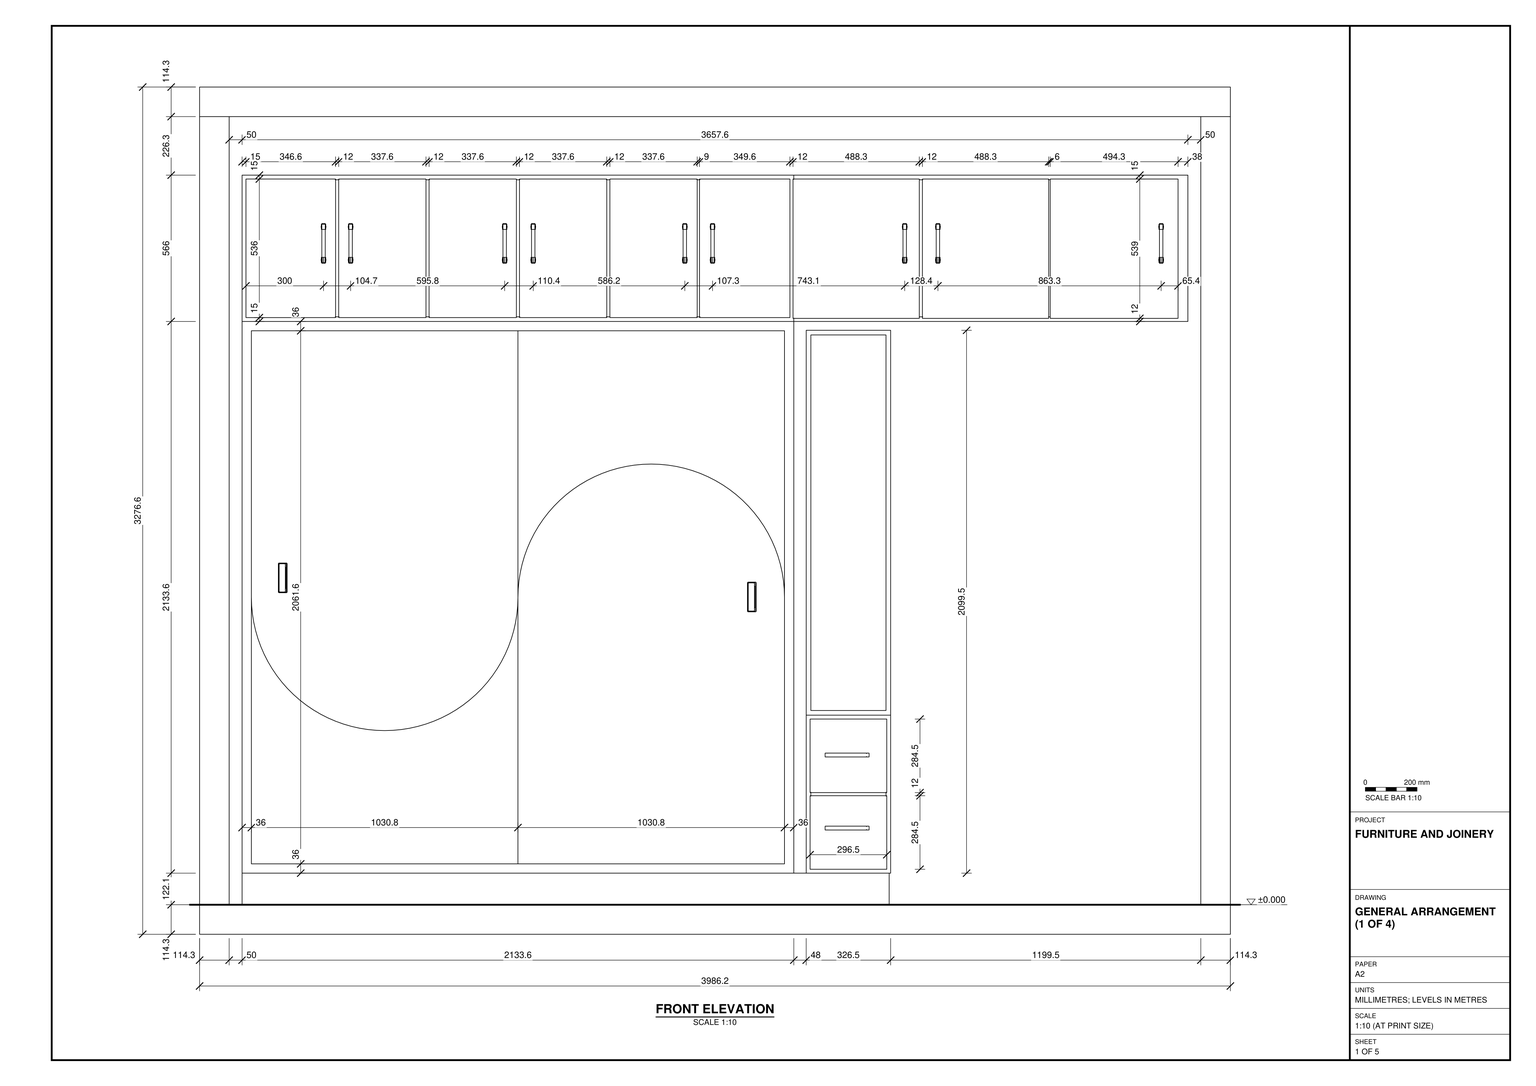
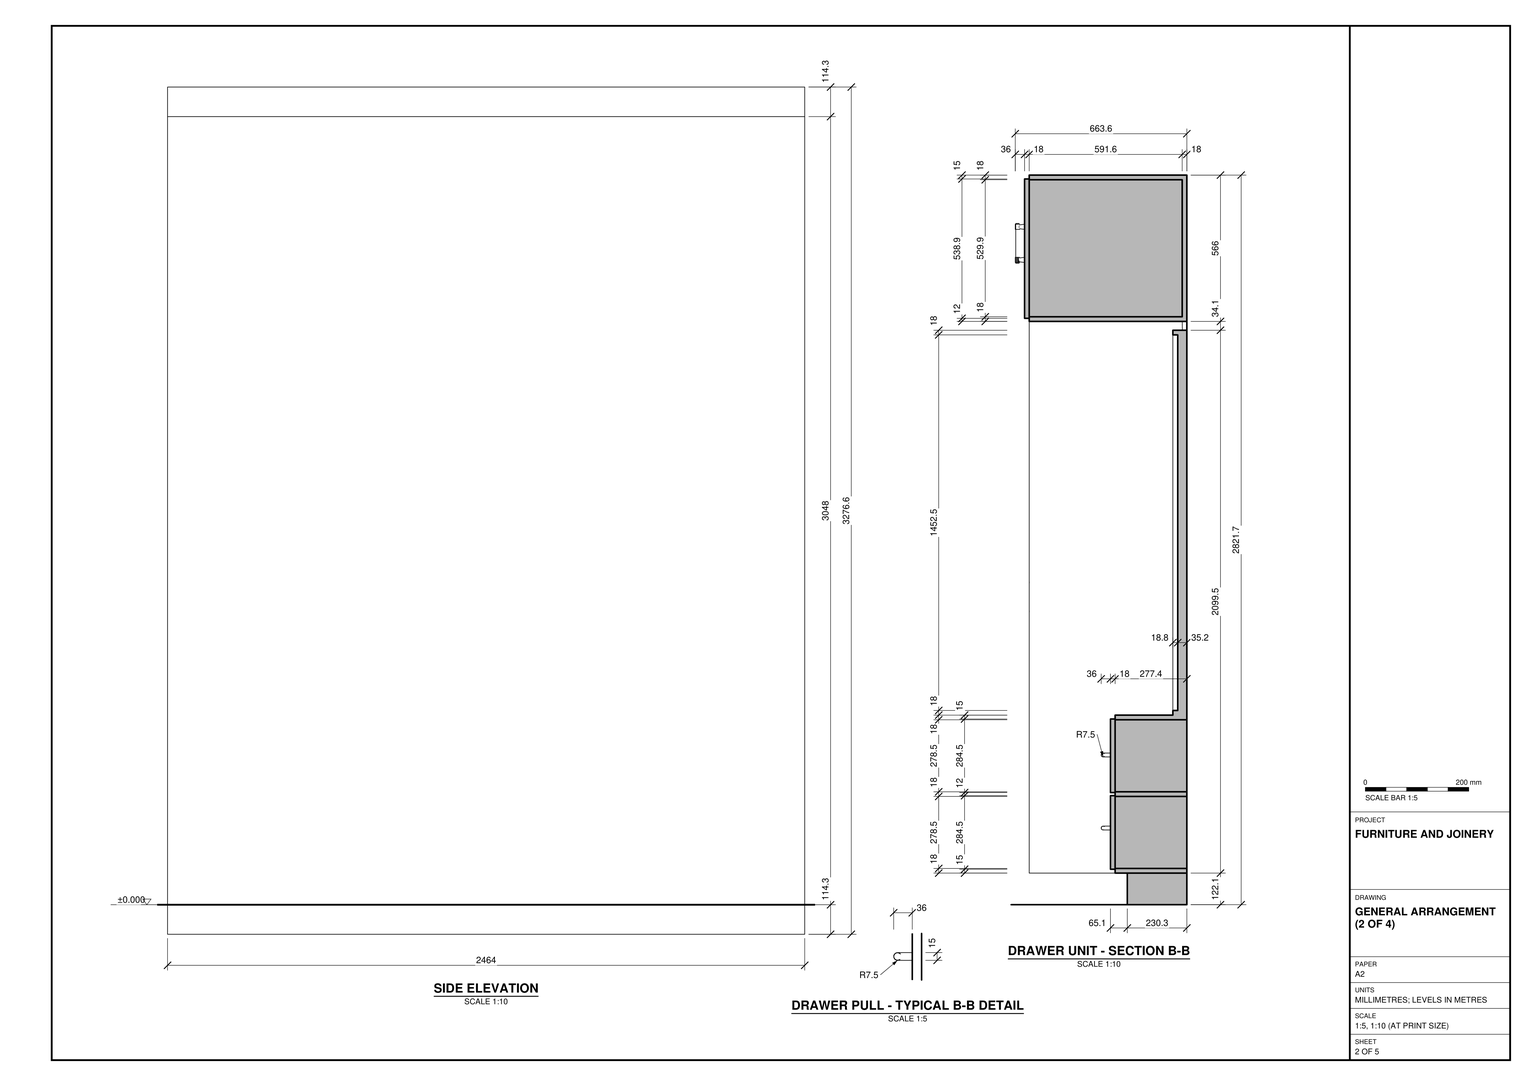
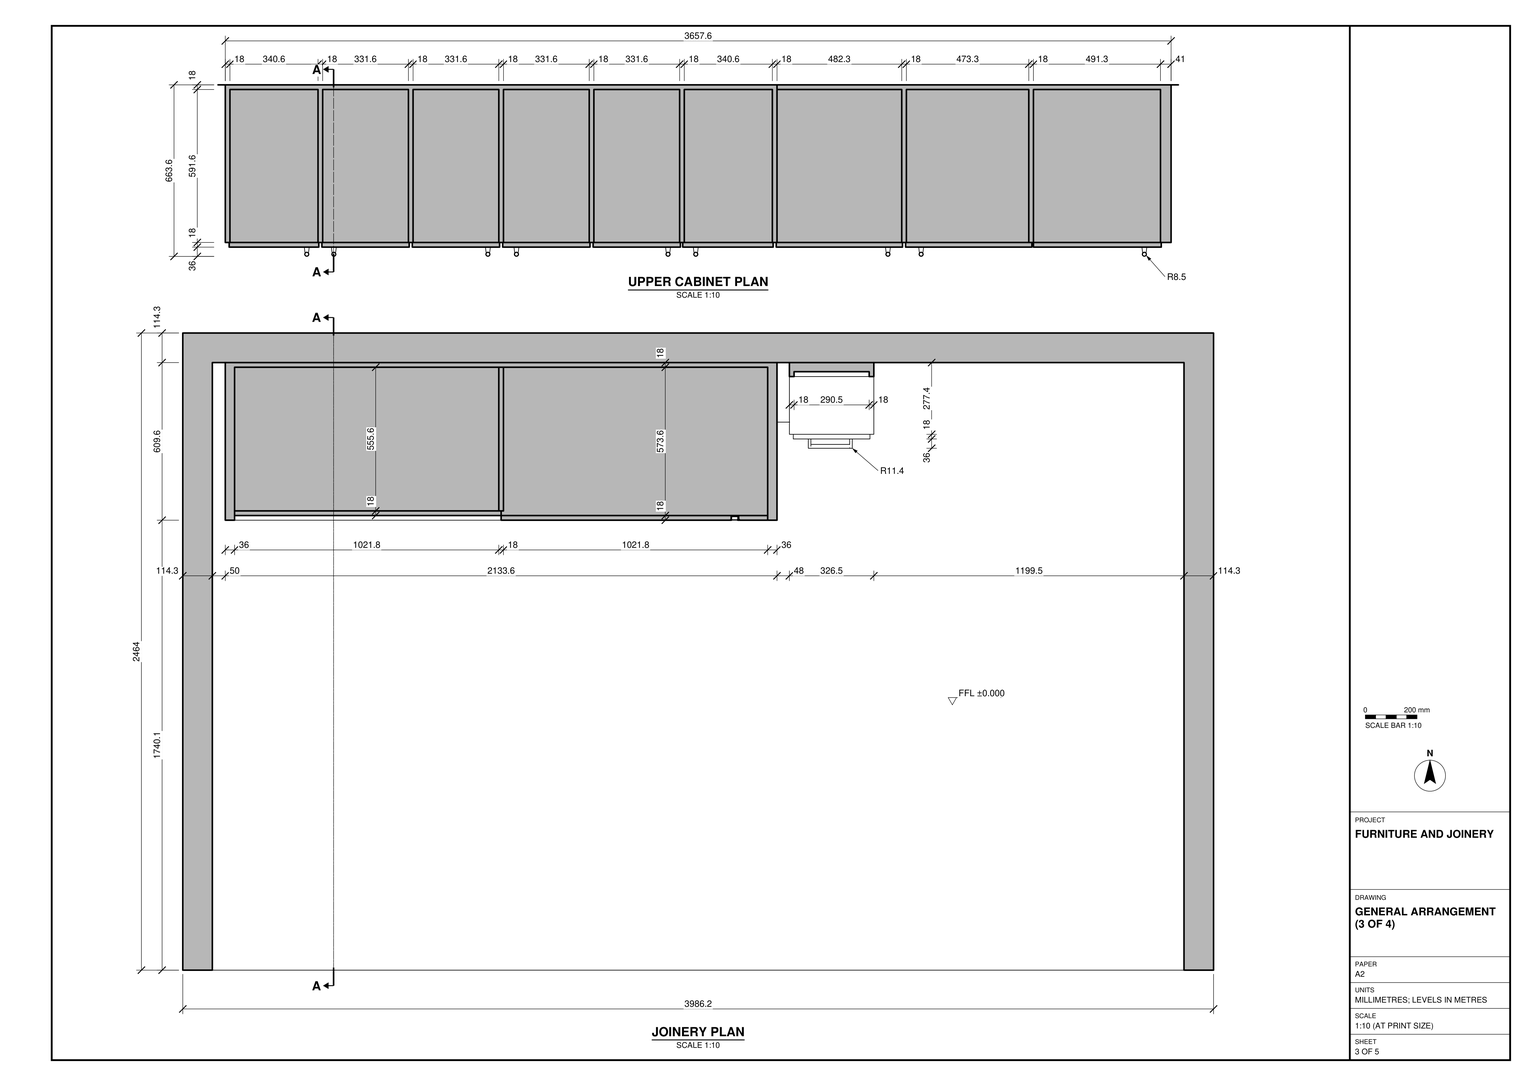
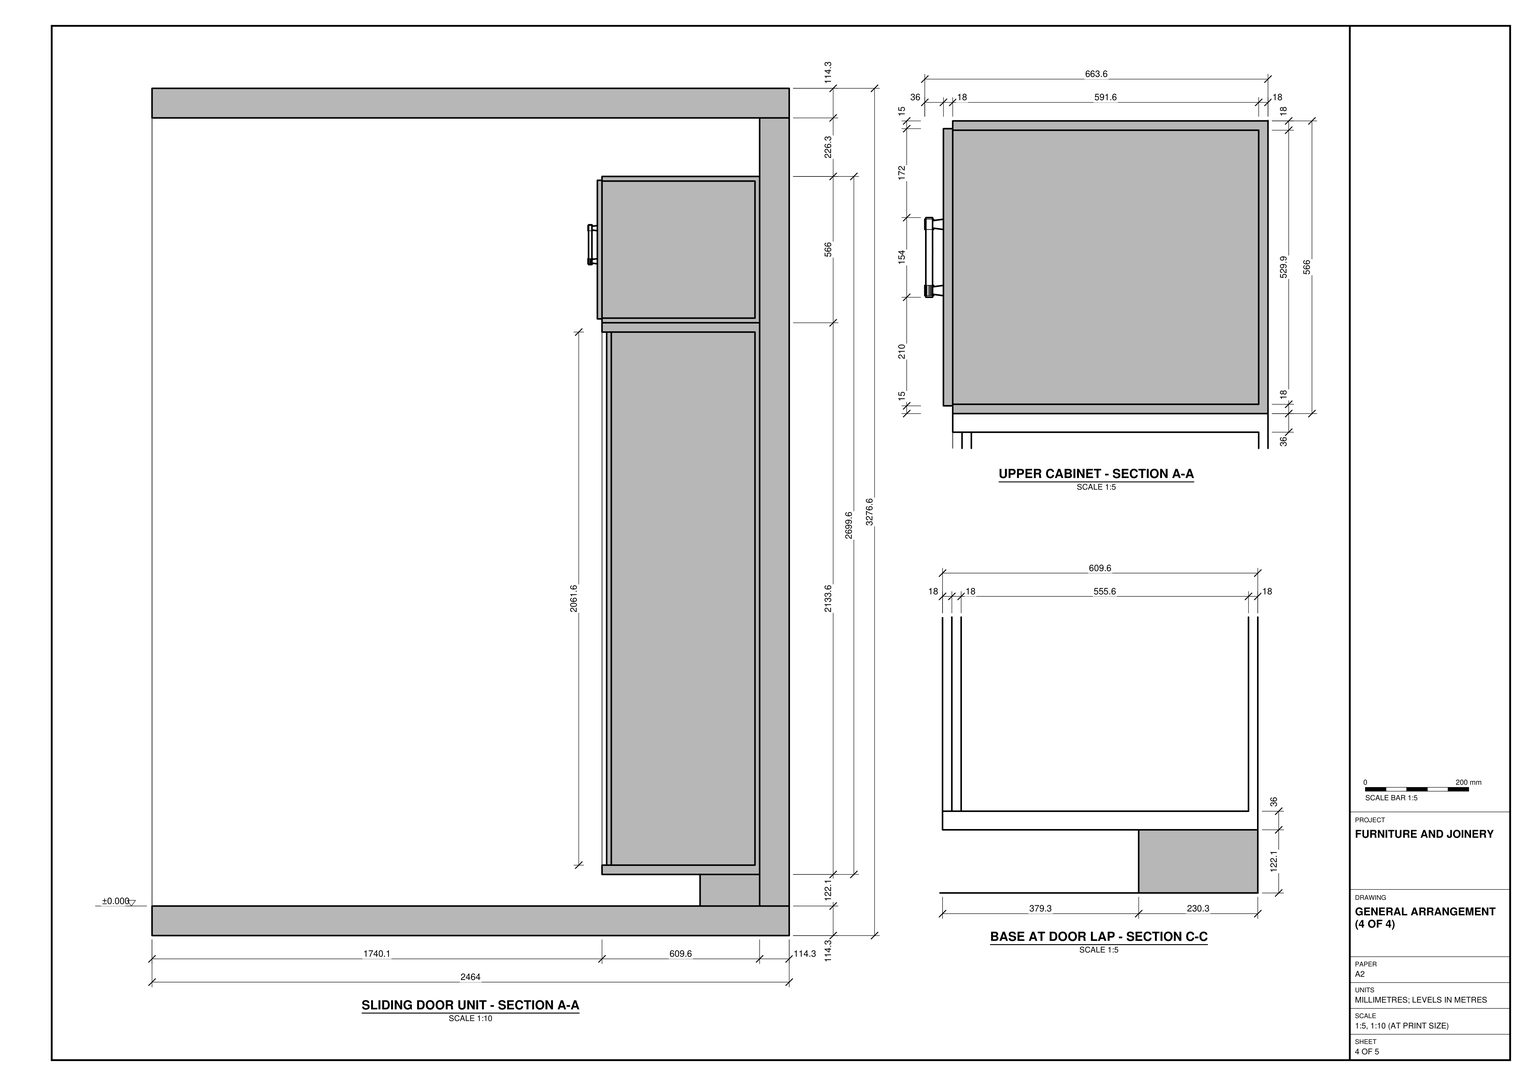
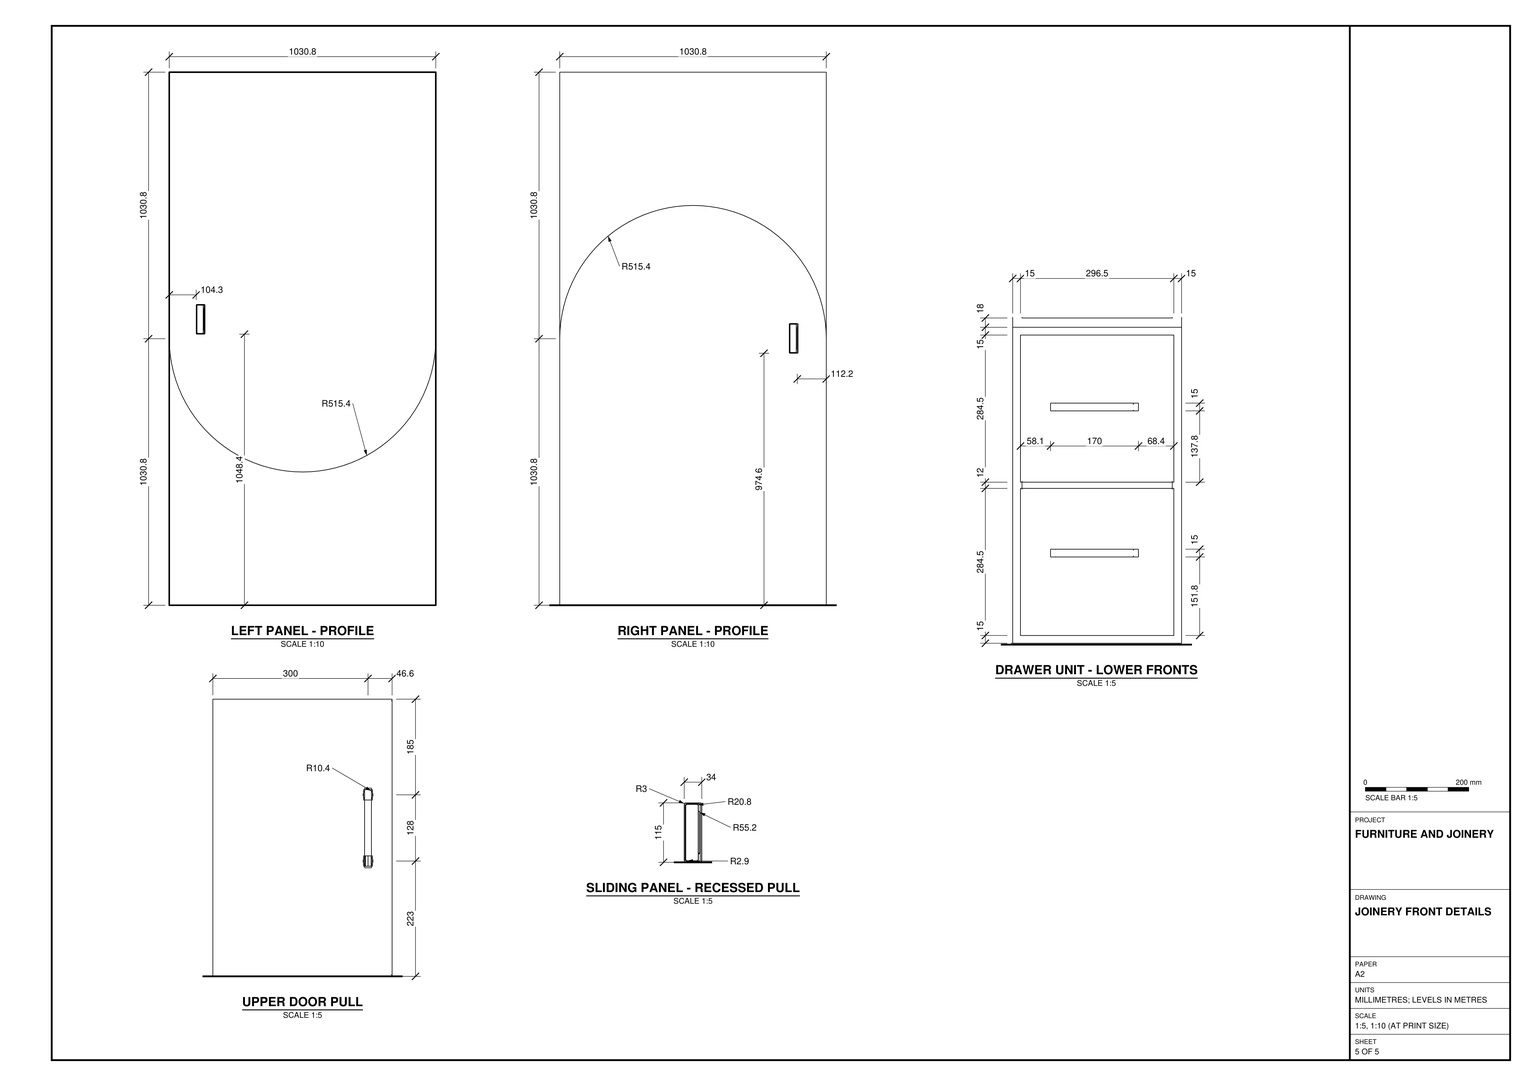
Work in millimetres in SketchUp using task_files/diagram_01.pdf. Model the wardrobe and its open-front enclosure, with an overall width of 3986.2 mm, depth of 2464 mm and height of 3276.6 mm. Use the finished floor as the single storey datum at 0 mm (±0.000). Include the floor slab, back wall, side walls and top slab at the 114.3 mm thickness shown.

Place the wardrobe against the back wall on the left. Build its carcass and plinth, then fit the two sliding fronts with the opposed curved outlines and inset pulls shown in elevation. To the right of the wardrobe, model the shallower drawer unit with horizontal pulls and a tall framed panel above it. Leave the space to its right open below the overhead cabinets. Extend the overhead run across all three areas, following the bay widths in plan and the door divisions and pull positions in elevation.

Keep the shell elements and each joinery piece in separate groups or components, and use components for repeated parts such as matching pulls. Any decor or loose items shown may be suitable library components. Save one SketchUp model as output_files/built_in_wardrobe_with_overhead_cabinets_and_drawers.skp.

# SketchUp Ruby script. Lengths in millimetres.
U = 1.mm
M = Sketchup.active_model
def pt(a) = Geom::Point3d.new(a.map { |v| v * U })
def face(e, loops, mat)
  f = e.add_face(loops[0].map { |a| pt(a) })
  loops[1..].each { |l| e.add_face(l.map { |a| pt(a) }).erase! }
  f.material = f.back_material = mat if mat
  f
end
# faces: each face lists its corners as indices into pts; further lists are holes
def faces(e, pts, list, mat = nil) = list.each { |f| face(e, (f[0].is_a?(Array) ? f : [f]).map { |l| l.map { |i| pts[i] } }, mat) }
# xy, xz, yz: faces in a plane at the given z, y or x. An outline is a flat list of corners, or four numbers for a rectangle; further outlines are holes
def ring(l) = l.size == 4 ? [[l[0], l[1]], [l[2], l[1]], [l[2], l[3]], [l[0], l[3]]] : l.each_slice(2).to_a
def flat(e, list, mat, &to3) = list.each { |f| face(e, (f[0].is_a?(Array) ? f : [f]).map { |l| ring(l).map { |u, v| to3.(u, v) } }, mat) }
def xy(e, z, list, mat = nil) = flat(e, list, mat) { |x, y| [x, y, z] }
def xz(e, y, list, mat = nil) = flat(e, list, mat) { |x, z| [x, y, z] }
def yz(e, x, list, mat = nil) = flat(e, list, mat) { |y, z| [x, y, z] }
def lines(e, pts, list) = list.each { |a, b| e.add_line(pt(pts[a]), pt(pts[b])) }
# prism: a flat outline (further loops are holes) pulled along v
def prism(e, loops, v, mat = nil)
  f = face(e, loops, mat); d = Geom::Vector3d.new(v.map { |x| x * U })
  f.pushpull(f.normal.samedirection?(d) ? d.length : -d.length)
end
def box(e, o, s, mat = nil) = prism(e, [[o, [o[0] + s[0], o[1], o[2]], [o[0] + s[0], o[1] + s[1], o[2]], [o[0], o[1] + s[1], o[2]]]], [0, 0, s[2]], mat)
def at(x, y, z, deg = 0) = Geom::Transformation.translation(pt([x, y, z])) * Geom::Transformation.rotation(ORIGIN, Z_AXIS, deg.degrees)
def axes(o, x, y, z) = Geom::Transformation.new([*x, 0, *y, 0, *z, 0, *pt(o).to_a, 1])
def part(name) = M.definitions.add(name)
# library, detail: a bought-in or finely detailed component or shape, given as its bounding box
def library(name, o, s) = part(name).tap { |d| box(d.entities, o, s) }
def detail(e, o, s) = box(e.add_group.entities, o, s)
def put(e, d, t, mat = nil) = e.add_instance(d, t).tap { |i| i.material = mat if mat }
def group(e, t, mat = nil) = e.add_group.tap { |g| g.transformation = t; g.material = mat if mat }.entities
root = M.entities
M.materials.add("[Color C04]").color = [255, 153, 50]
M.materials.add("[Color K02]").color = [255, 153, 255]
M.materials.add("[Color L04]").color = [255, 50, 152]
M.materials.add("[Formica Beige]").color = [211, 187, 149]
M.materials.add("[Marble Carrara Gold Floor Tile]").color = [225, 223, 217]
M.materials.add("[Translucent Glass Blue]").color = [100, 149, 237]
M.materials["[Translucent Glass Blue]"].alpha = 0.5
M.materials.add("[Wood Bamboo]").color = [177, 105, 43]
M.materials.add("[Wood Veneer 01]").color = [120, 70, 37]
c1 = part("Overhead cabinet door")
g1 = group(c1.entities,at(-3,-18,-3))
box(g1,[0,0,0],[337.6,18,535.9])
c2 = part("Overhead cabinet door \#1")
box(c2.entities,[-3,-18,-3],[337.6,18,535.9])
c3 = part("Overhead cabinet door \#2")
box(c3.entities,[-3,-18,-3],[337.6,18,535.9])
c4 = part("Overhead cabinet door \#3")
box(c4.entities,[-3,-18,-3],[337.6,18,535.9])
c5 = library("1-POIGNEE CLC2",[-77,-9.5,0],[154,19,36])
c6 = library("6-POIGNEE CLC2",[-85,-7.5,0],[170,15,36])
c7 = library("Group\#17",[0,-18,0],[1030.8,18,2061.6])
c8 = library("Group\#4",[0,-18,0],[1030.8,18,2061.6])
xy(root,926.5,[[164.3,2119.4,2666.7,2349.7]],"[Color C04]")
xy(root,926.5,[[0,0,114.3,2464],[3871.9,0,3986.2,2464],[114.3,2349.7,164.3,2464],[164.3,2349.7,3871.9,2464]],"[Formica Beige]")
xy(root,1048.6,[[164.3,2119.4,2297.9,2349.7],[2297.9,2119.4,2666.7,2349.7]])
xy(root,3974.5,[[0,0,114.3,0,114.3,2349.7,3871.9,2349.7,3871.9,0,3986.2,0,3986.2,2464,0,2464]],"[Formica Beige]")
xz(root,0,[[0,926.5,114.3,3974.5],[3871.9,926.5,3986.2,3974.5]],"[Formica Beige]")
xz(root,2119.4,[[164.3,926.5,2666.7,1048.6]],"[Color C04]")
xz(root,2349.7,[[164.3,926.5,2666.7,1048.6]])
xz(root,2349.7,[[114.3,926.5,164.3,926.5,164.3,1048.6,2666.7,1048.6,2666.7,926.5,3871.9,926.5,3871.9,3974.5,114.3,3974.5]],"[Formica Beige]")
xz(root,2464,[[0,926.5,3871.9,3974.5],[3871.9,926.5,3986.2,3974.5]],"[Formica Beige]")
yz(root,0,[[0,926.5,2464,3974.5]],"[Formica Beige]")
yz(root,114.3,[[0,926.5,2349.7,3974.5]],"[Formica Beige]")
yz(root,164.3,[[2119.4,926.5,2349.7,1048.6]],"[Color C04]")
yz(root,2666.7,[[2119.4,926.5,2349.7,1048.6]],"[Color C04]")
yz(root,3871.9,[[0,926.5,2349.7,3974.5]],"[Formica Beige]")
yz(root,3986.2,[[0,926.5,2464,3974.5]],"[Formica Beige]")
p = [[2297.9,2349.7,1048.6],[2297.9,2331.7,3200.2],[2796.9,2331.7,3200.2]]
lines(root,p,[[0,1],[1,2]])
put(root,c1,at(540.9,1740.1,3200.2))
put(root,c2,at(890.5,1740.1,3200.2))
put(root,c3,at(1240.1,1740.1,3200.2))
put(root,c4,at(1589.7,1740.1,3200.2))
put(root,c5,axes([479.3,1722.1,3484.2],[0,0,1],[-1,0,0],[0,-1,0]))
put(root,c5,axes([584.1,1722.1,3484.2],[0,0,1],[-1,0,0],[0,-1,0]))
put(root,c5,axes([1179.8,1722.1,3484.2],[0,0,1],[-1,0,0],[0,-1,0]))
put(root,c5,axes([1290.2,1722.1,3484.2],[0,0,1],[-1,0,0],[0,-1,0]))
put(root,c5,axes([1876.4,1722.1,3484.2],[0,0,1],[-1,0,0],[0,-1,0]))
put(root,c5,axes([1983.7,1722.1,3484.2],[0,0,1],[-1,0,0],[0,-1,0]))
put(root,c5,axes([2726.8,1722.1,3484.2],[0,0,1],[-1,0,0],[0,-1,0]))
put(root,c5,axes([2855.2,1722.1,3484.2],[0,0,1],[-1,0,0],[0,-1,0]))
put(root,c5,axes([3718.5,1722.1,3484.2],[0,0,1],[-1,0,0],[0,-1,0]))
put(root,c6,axes([2504,2054.3,1505.4],[1,0,0],[0,0,1],[0,-1,0]))
put(root,c6,axes([2504,2054.3,1223],[1,0,0],[0,0,1],[0,-1,0]),"[Color K02]")
g2 = group(root,at(182.3,1740.1,3200.2))
box(g2,[-3,-18,-3],[346.6,18,535.9])
g3 = group(root,at(1939.3,1740.1,3200.2))
box(g3,[-6,-18,-3],[349.6,18,535.9])
g4 = group(root,at(2303.9,1740.1,3197.2))
box(g4,[-9,-18,-3],[488.3,18,538.9])
g5 = group(root,at(2804.2,1740.1,3197.2))
box(g5,[-9,-18,-3],[488.3,18,538.9])
g6 = group(root,at(3295.6,1740.1,3197.2))
box(g6,[-6,-18,-3],[494.3,18,538.9])
g7 = group(root,at(164.3,1740.1,3182.2),"[Wood Bamboo]")
xy(g7,0,[[0,0,2133.6,609.6],[2133.6,0,3657.6,609.6]])
xy(g7,18,[[18,0,358.6,591.6],[376.6,0,708.2,591.6],[726.2,0,1057.8,591.6],[1075.8,0,1407.4,591.6],[1425.4,0,1757,591.6],
  [1775,0,2115.6,591.6],[2133.6,0,2615.9,591.6],[2633.9,0,3107.3,591.6],[3125.3,0,3616.6,591.6]])
xy(g7,547.9,[[18,0,358.6,591.6],[376.6,0,708.2,591.6],[726.2,0,1057.8,591.6],[1075.8,0,1407.4,591.6],[1425.4,0,1757,591.6],
  [1775,0,2115.6,591.6],[2133.6,0,2615.9,591.6],[2633.9,0,3107.3,591.6],[3125.3,0,3616.6,591.6]])
xy(g7,565.9,[[0,0,2133.6,609.6],[2133.6,0,3657.6,609.6]])
xz(g7,0,[[[0,0,2133.6,565.9],[18,18,2115.6,547.9]],[2133.6,0,3657.6,0,3657.6,565.9,2133.6,565.9,2133.6,547.9,3616.6,547.9,3616.6,18,2133.6,18],[358.6,18,376.6,547.9],[708.2,18,726.2,547.9],[1057.8,18,1075.8,547.9],
  [1407.4,18,1425.4,547.9],[1757,18,1775,547.9],[2615.9,18,2633.9,547.9],[3107.3,18,3125.3,547.9]])
xz(g7,591.6,[[18,18,358.6,547.9],[376.6,18,708.2,547.9],[726.2,18,1057.8,547.9],[1075.8,18,1407.4,547.9],[1425.4,18,1757,547.9],
  [1775,18,2115.6,547.9],[2133.6,18,2615.9,547.9],[2633.9,18,3107.3,547.9],[3125.3,18,3616.6,547.9]])
xz(g7,609.6,[[0,0,2133.6,565.9],[2133.6,0,3657.6,565.9]])
yz(g7,0,[[0,0,609.6,565.9]])
yz(g7,18,[[0,18,591.6,547.9]])
yz(g7,358.6,[[0,18,591.6,547.9]])
yz(g7,376.6,[[0,18,591.6,547.9]])
yz(g7,708.2,[[0,18,591.6,547.9]])
yz(g7,726.2,[[0,18,591.6,547.9]])
yz(g7,1057.8,[[0,18,591.6,547.9]])
yz(g7,1075.8,[[0,18,591.6,547.9]])
yz(g7,1407.4,[[0,18,591.6,547.9]])
yz(g7,1425.4,[[0,18,591.6,547.9]])
yz(g7,1757,[[0,18,591.6,547.9]])
yz(g7,1775,[[0,18,591.6,547.9]])
yz(g7,2115.6,[[0,18,591.6,547.9]])
yz(g7,2133.6,[[0,0,0,18,591.6,18,591.6,547.9,0,547.9,0,565.9,609.6,565.9,609.6,0],[0,18,591.6,547.9]])
yz(g7,2615.9,[[0,18,591.6,547.9]])
yz(g7,2633.9,[[0,18,591.6,547.9]])
yz(g7,3107.3,[[0,18,591.6,547.9]])
yz(g7,3125.3,[[0,18,591.6,547.9]])
yz(g7,3616.6,[[0,18,591.6,547.9]])
yz(g7,3657.6,[[0,0,609.6,565.9]])
g8 = group(root,at(2345.9,2349.7,1048.6))
xy(g8,0,[[0,-277.4,326.5,0]],"[Wood Veneer 01]")
xy(g8,18,[[18,-277.4,308.5,0]],"[Wood Veneer 01]")
xy(g8,296.5,[[18,-277.4,308.5,0]],"[Wood Veneer 01]")
xy(g8,314.5,[[18,-277.4,308.5,0]],"[Wood Veneer 01]")
xy(g8,593,[[18,-277.4,308.5,0]],"[Wood Veneer 01]")
xy(g8,611,[[0,-277.4,326.5,-54.1]],"[Wood Veneer 01]")
xy(g8,629,[[18,-54.1,308.5,-35.2]],"[Wood Veneer 01]")
xy(g8,2081.5,[[18,-54.1,308.5,-35.2]],"[Wood Veneer 01]")
xy(g8,2099.5,[[0,-54.1,326.5,0]],"[Wood Veneer 01]")
xz(g8,-277.4,[[[0,0,326.5,611],[18,18,308.5,593]],[18,296.5,308.5,314.5]],"[Wood Veneer 01]")
xz(g8,-54.1,[[[0,611,326.5,2099.5],[18,629,308.5,2081.5]]],"[Wood Veneer 01]")
xz(g8,-35.2,[[18,629,308.5,2081.5]],"[Translucent Glass Blue]")
xz(g8,0,[[18,18,308.5,296.5],[18,314.5,308.5,593]],"[Wood Veneer 01]")
yz(g8,0,[[-277.4,0,0,611],[-54.1,611,0,2099.5]],"[Wood Veneer 01]")
yz(g8,18,[[-277.4,18,0,296.5],[-277.4,314.5,0,593],[-54.1,629,-35.2,2081.5]],"[Wood Veneer 01]")
yz(g8,308.5,[[-277.4,18,0,296.5],[-277.4,314.5,0,593],[-54.1,629,-35.2,2081.5]],"[Wood Veneer 01]")
yz(g8,326.5,[[-277.4,0,0,611],[-54.1,611,0,2099.5]],"[Wood Veneer 01]")
g9 = group(root,at(2363.9,2072.3,1363.1),"[Color L04]")
box(g9,[-3,-18,-3],[296.5,18,284.5])
g10 = group(root,at(2363.9,2072.3,1066.6),"[Color L04]")
box(g10,[-3,-18,-3],[296.5,18,284.5])
g11 = group(root,at(114.3,0,3974.5))
box(g11,[-114.3,0,0],[3986.2,2464,114.3])
g12 = group(root,at(114.3,0,812.2))
xy(g12,0,[[-114.3,0,3871.9,2464]])
xy(g12,114.3,[[-114.3,0,3871.9,2464]],"[Marble Carrara Gold Floor Tile]")
xz(g12,0,[[-114.3,0,3871.9,114.3]])
xz(g12,2464,[[-114.3,0,3871.9,114.3]])
yz(g12,-114.3,[[0,0,2464,114.3]])
yz(g12,3871.9,[[0,0,2464,114.3]])
g13 = group(root,at(164.3,1740.1,1048.6),"[Wood Bamboo]")
xy(g13,0,[[0,0,2133.6,609.6]])
xy(g13,36,[[36,0,2097.6,591.6]])
xy(g13,2097.6,[[36,0,2097.6,591.6]])
xy(g13,2133.6,[[0,0,2133.6,609.6]])
xz(g13,0,[[[0,0,2133.6,2133.6],[36,36,2097.6,2097.6]]])
xz(g13,591.6,[[1075.8,36,2097.6,2097.6]])
xz(g13,609.6,[[0,0,2133.6,2133.6]])
yz(g13,0,[[0,0,609.6,2133.6]])
yz(g13,36,[[0,36,36,2097.6],[36,36,591.6,2097.6]])
yz(g13,2097.6,[[0,36,591.6,2097.6]])
yz(g13,2133.6,[[0,0,609.6,2133.6]])
g14 = group(g13,at(1057.8,591.6,36))
box(g14,[0,-555.6,0],[18,555.6,2061.6])
g15 = group(g13,at(36,591.6,36))
xz(g15,0,[[0,0,1021.8,2061.6]])
put(g13,c7,at(36,36,36))
put(g13,c8,axes([1066.8,18,2097.6],[1,0,0],[0,1,0],[0,0,-1]))
